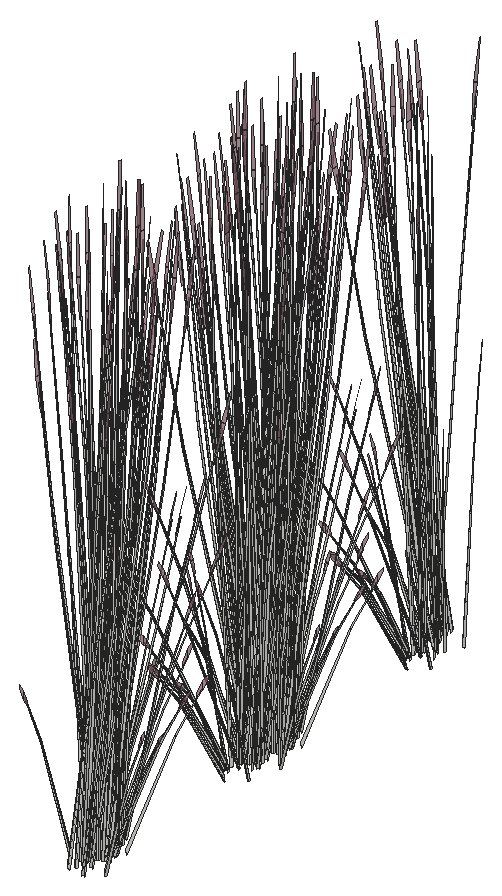
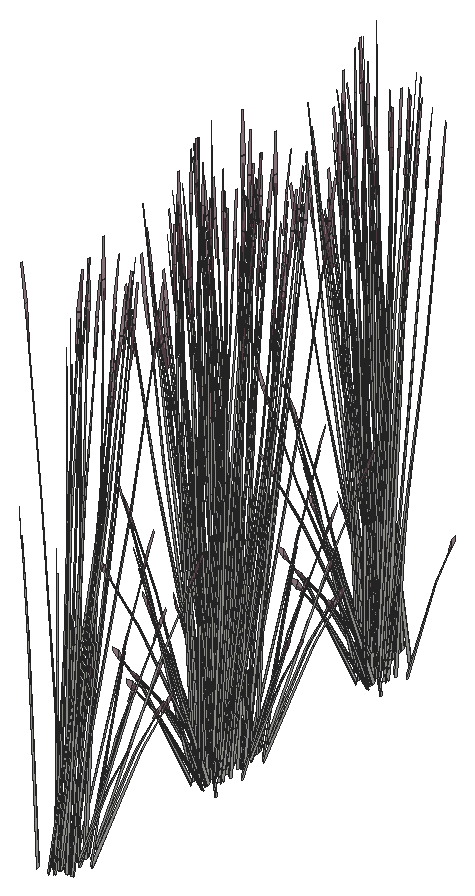
# SketchUp Ruby script. Lengths in inches.
U = 1.inch
M = Sketchup.active_model
def pt(a) = Geom::Point3d.new(a.map { |v| v * U })
def face(e, loops, mat)
  f = e.add_face(loops[0].map { |a| pt(a) })
  loops[1..].each { |l| e.add_face(l.map { |a| pt(a) }).erase! }
  f.material = f.back_material = mat if mat
  f
end
# faces: each face lists its corners as indices into pts; further lists are holes
def faces(e, pts, list, mat = nil) = list.each { |f| face(e, (f[0].is_a?(Array) ? f : [f]).map { |l| l.map { |i| pts[i] } }, mat) }
# xy, xz, yz: faces in a plane at the given z, y or x. An outline is a flat list of corners, or four numbers for a rectangle; further outlines are holes
def ring(l) = l.size == 4 ? [[l[0], l[1]], [l[2], l[1]], [l[2], l[3]], [l[0], l[3]]] : l.each_slice(2).to_a
def flat(e, list, mat, &to3) = list.each { |f| face(e, (f[0].is_a?(Array) ? f : [f]).map { |l| ring(l).map { |u, v| to3.(u, v) } }, mat) }
def xy(e, z, list, mat = nil) = flat(e, list, mat) { |x, y| [x, y, z] }
def xz(e, y, list, mat = nil) = flat(e, list, mat) { |x, z| [x, y, z] }
def yz(e, x, list, mat = nil) = flat(e, list, mat) { |y, z| [x, y, z] }
def lines(e, pts, list) = list.each { |a, b| e.add_line(pt(pts[a]), pt(pts[b])) }
# prism: a flat outline (further loops are holes) pulled along v
def prism(e, loops, v, mat = nil)
  f = face(e, loops, mat); d = Geom::Vector3d.new(v.map { |x| x * U })
  f.pushpull(f.normal.samedirection?(d) ? d.length : -d.length)
end
def box(e, o, s, mat = nil) = prism(e, [[o, [o[0] + s[0], o[1], o[2]], [o[0] + s[0], o[1] + s[1], o[2]], [o[0], o[1] + s[1], o[2]]]], [0, 0, s[2]], mat)
def at(x, y, z, deg = 0) = Geom::Transformation.translation(pt([x, y, z])) * Geom::Transformation.rotation(ORIGIN, Z_AXIS, deg.degrees)
def axes(o, x, y, z) = Geom::Transformation.new([*x, 0, *y, 0, *z, 0, *pt(o).to_a, 1])
def part(name) = M.definitions.add(name)
# library, detail: a bought-in or finely detailed component or shape, given as its bounding box
def library(name, o, s) = part(name).tap { |d| box(d.entities, o, s) }
def detail(e, o, s) = box(e.add_group.entities, o, s)
def put(e, d, t, mat = nil) = e.add_instance(d, t).tap { |i| i.material = mat if mat }
def group(e, t, mat = nil) = e.add_group.tap { |g| g.transformation = t; g.material = mat if mat }.entities
root = M.entities
M.materials.add("LightPink_Translucent").color = [144, 107, 117]
M.materials["LightPink_Translucent"].alpha = 0.75
c1 = part("blade")
p = [[2.15,0.21,22],[0,0.17,0],[0.09,0.45,0],[2.18,0.31,22],[2.29,0.31,22],[0.38,0.45,0],
  [2.48,0.24,33],[2.49,0.24,33],[2.48,0.22,33]]
faces(c1.entities,p,[[0,1,2,3],[4,5,2,3],[6,3,4,7],[8,0,3,6]])
c2 = part("seeds")
p = [[0.3,-0.1,1.38],[-0.01,-0.03,1.59],[-0.01,-0.03,0.03],[0.14,-0.07,-0.07],[0.29,-0.03,3],[0.15,0.01,3.11]]
faces(c2.entities,p,[[0,1,2,3],[1,0,4,5]],"LightPink_Translucent")
c3 = part("blade with seeds")
put(c3.entities,c1,at(0,0,0))
put(c3.entities,c2,axes([2.4,0.25,30.99],[1.5799,-0.05474,1.17369],[-0.12525,1.92788,0.29478],[-0.07173,-0.02425,1.56792]))
put(root,c3,axes([251.23,97.13,0.35],[-0.25194,0.2448,0.93574],[-0.08019,-0.7024,0.36359],[0.1547,0.01169,1.0643]))
put(root,c3,axes([251.91,97.3125,1.09],[0.04938,-0.54569,0.10509],[0.24125,0.09472,-0.30009],[0.0439,0.05603,0.91989]))
put(root,c3,axes([251.49,98.61,0.91],[0.32351,0.12883,0.33208],[-0.06584,0.72759,0.13031],[-0.04728,-0.07026,1.15295]))
put(root,c3,axes([253.2,98.08,0.28],[-0.01338,-0.09283,1.27986],[0.09278,-0.54301,-0.19552],[0.09359,-0.00781,0.218]))
put(root,c3,axes([250.44,97.99,0.28],[0.00649,0.09636,1.27986],[-0.13086,0.50324,-0.19552],[-0.09295,-0.02537,0.218]))
put(root,c3,axes([251.81,97.46,1.17],[-0.15376,-0.51322,0.32471],[0.2329,-0.3614,-0.15627],[0.04976,0.0635,1.04254]))
put(root,c3,axes([251.01,99.8,0.66],[-0.06012,-0.53279,-0.22483],[0.23879,-0.15129,0.22483],[-0.04814,-0.06144,1.00865]))
put(root,c3,axes([251.32,99.77,0.99],[0.27504,-0.16229,0.12804],[0.06792,0.60396,0.25465],[-0.02453,-0.088,1.1642]))
put(root,c3,axes([251.89,97.49,1.13],[0.25843,-0.40595,-0.21117],[0.17185,0.5736,-0.36291],[0.06376,0.05825,1.15913]))
put(root,c3,axes([250.95,100.03,0.66],[-0.23955,-0.30573,-0.36036],[0.14318,-0.54821,0],[-0.05456,-0.06963,1.14313]))
put(root,c3,axes([252.54,96.41,0.66],[0.23955,0.30573,-0.36036],[-0.14318,0.54821,0],[0.05456,0.06963,1.14313]))
put(root,c3,axes([252.08,98.16,0.79],[0.28637,0,0],[0,0.63302,0],[0,0,1.29484]))
put(root,c3,axes([251.6,98.95,1.13],[-0.25843,0.40595,-0.21117],[-0.17185,-0.5736,-0.36291],[-0.06376,-0.05825,1.15913]))
put(root,c3,axes([252.16,96.67,0.99],[-0.27504,0.16229,0.12804],[-0.06792,-0.60396,0.25465],[0.02453,0.088,1.1642]))
put(root,c3,axes([252.47,96.64,0.66],[0.06012,0.53279,-0.22483],[-0.23879,0.15129,0.22483],[0.04814,0.06144,1.00865]))
put(root,c3,axes([251.99,97.83,0.92],[-0.32351,-0.12883,0.35707],[0.06584,-0.72759,0.14012],[0.04728,0.07026,1.23973]))
put(root,c3,axes([251.73,99.63,0.79],[-0.08351,-0.52716,0],[0.23848,-0.18461,0],[0,0,1.1204]))
put(root,c3,axes([251.57,99.13,1.09],[-0.04938,0.54569,0.10509],[-0.24125,-0.09472,-0.30009],[-0.0439,-0.05603,0.91989]))
put(root,c3,axes([252.05,99.56,0.78],[0.26872,-0.20746,-0.13933],[0.09442,0.59762,0.00006],[0.02966,-0.02293,1.26212]))
put(root,c3,axes([252.14,99.8,0.99],[0.07394,-0.60768,0.12804],[0.27057,0.17197,0.25465],[-0.04674,0.00296,1.1642]))
put(root,c3,axes([252.08,98.43,0.8],[0.17867,0.39495,0],[-0.17867,0.39495,0],[0,0,1.22851]))
put(root,c3,axes([252.5625,98.25,0.99],[-0.2011,-0.44539,0.12804],[0.20266,-0.432,0.25465],[-0.02221,0.09096,1.1642]))
put(root,c3,axes([252.1875,97.58,0.6875],[0.26625,0.10025,-0.45255],[-0.05619,0.61836,-0.11877],[0.07946,0.07493,0.99892]))
put(root,c3,axes([253.36,98.66,1.2],[-0.15814,0.10094,0.83364],[0.07444,-0.41719,0.6125],[0.0839,0.02855,0.18362]))
put(root,c3,axes([251.67,99.87,0.79],[-0.25804,-0.27452,0],[0.12419,-0.5704,0],[0,0,1.1809]))
put(root,c3,axes([251.89,99.14,0.98],[-0.24993,-0.49214,-0.18284],[0.21031,-0.55263,0.40012],[-0.0673,0.05757,1.22088]))
put(root,c3,axes([251.23,100.08,0.99],[0.23955,0.30573,0.36036],[-0.14318,0.54821,0],[-0.05456,-0.06963,1.14313]))
put(root,c3,axes([252.07,97.96,1.17],[0.12419,-0.55096,0.32471],[0.25804,0.26516,-0.15627],[0,0.12701,1.04254]))
put(root,c3,axes([252.03,98.28,0.86],[0,0.70714,-0.04091],[-0.32006,0,0],[0,0.02222,1.30182]))
put(root,c3,axes([252.05,97.78,0.8],[0.15376,0.51322,-0.32471],[-0.2329,0.3614,0.15627],[0.04976,0.0635,1.04254]))
put(root,c3,axes([251.09,100.4,0.91],[-0.16003,0.61271,0],[-0.26773,-0.34169,-0.37456],[-0.06098,-0.07782,1.18819]))
put(root,c3,axes([252.73,98.27,0.99],[0,-0.61145,0.36036],[0.28637,0,0],[0,0.13926,1.14313]))
put(root,c3,axes([252.01,98.73,1.17],[0.27795,-0.03775,0.32471],[0.02514,0.62656,-0.15627],[-0.04976,0.0635,1.04254]))
put(root,c3,axes([252.18,98.09,1.09],[0.23848,-0.17832,0.10509],[0.08351,0.5092,-0.30009],[0,0.11207,0.91989]))
put(root,c3,axes([251.76,99.03,0.8],[-0.27795,0.03775,-0.32471],[-0.02514,-0.62656,0.15627],[-0.04976,0.0635,1.04254]))
put(root,c3,axes([253.07,99.33,1.07],[-0.06164,-0.15038,1.03788],[0.0802,-0.49748,-0.22321],[0.12472,0.06739,0.44375]))
put(root,c3,axes([251.97,99.88,0.79],[0.25804,0.27452,0],[-0.12419,0.5704,0],[0,0,1.26978]))
put(root,c3,axes([252.07,100.49,0.78],[-0.15803,-0.61485,-0.03732],[0.26773,-0.34169,0.37456],[-0.06597,0.05854,1.1876]))
put(root,c3,axes([252.01,99,1.09],[0.1891,0.36737,0.10509],[-0.15773,0.41447,-0.30009],[-0.0439,0.05603,0.91989]))
put(root,c3,axes([252.21,100.13,0.99],[0.23955,-0.30573,0.36036],[0.14318,0.54821,0],[-0.05456,0.06963,1.14313]))
put(root,c3,axes([251.875,99.65,0.86],[0.11128,0.70245,-0.04364],[-0.31797,0.24614,0],[0.00389,0.02453,1.2496]))
put(root,c3,axes([252,100.41,0.66],[-0.23879,-0.15129,-0.22483],[0.06012,-0.53279,0.22483],[-0.04814,0.06144,1.00865]))
put(root,c3,axes([250.27,99.33,1.07],[0.08895,0.05019,1.03788],[0.05733,0.5127,-0.22321],[-0.12083,0.09597,0.44375]))
put(root,c3,axes([252.92,98.375,0.92],[0.32006,0,0],[0,0.68339,-0.37456],[0,0.15565,1.18819]))
put(root,c3,axes([252.79,98.73,0.79],[-0.3199,-0.00489,-0.03612],[0,-0.68339,0.36248],[-0.01005,0.15557,1.14929]))
put(root,c3,axes([252.1,98.13,1.13],[0.28825,0.29175,-0.21117],[-0.1388,0.61578,-0.36291],[0.00906,0.15119,1.15913]))
put(root,c3,axes([250.09,100.4,1.2],[0.10667,-0.27712,0.83364],[0.04209,0.43871,0.6125],[-0.07709,0.07855,0.18362]))
put(root,c3,axes([252.73,98.83,0.66],[-0.17867,0.3815,-0.22483],[-0.17867,-0.3815,0.22483],[0,0.12288,1.00865]))
put(root,c3,axes([251.96,98.86,1.13],[0.02983,0.6977,-0.21117],[-0.31064,0.04219,-0.36291],[-0.0547,0.09294,1.15913]))
put(root,c3,axes([252.07,98.59,0.8],[-0.12419,0.55096,-0.32471],[-0.25804,-0.26516,0.15627],[0,0.12701,1.04254]))
put(root,c3,axes([251.77,99.4,0.6875],[-0.1724,0.45959,-0.45255],[-0.21416,-0.41674,-0.11877],[-0.06908,0.11465,0.99892]))
put(root,c3,axes([252.08,100.17,0.88],[0.32044,0.19874,0.22322],[-0.08017,0.71038,-0.26485],[-0.05304,0.08891,1.19671]))
put(root,c3,axes([252.05,100.65,0.66],[-0.23955,0.30573,-0.36036],[-0.14318,-0.54821,0],[-0.05456,0.06963,1.14313]))
put(root,c3,axes([252.85,98.84,0.66],[0,0.61145,-0.36036],[-0.28637,0,0],[0,0.13926,1.14313]))
put(root,c3,axes([252.49,100.11,1.2],[-0.14411,-0.17581,0.83364],[0.18609,-0.17864,0.6125],[0.05019,0.15132,0.18362]))
put(root,c3,axes([252.27,100.55,0.91],[0.16003,0.61271,0],[-0.26773,0.34169,-0.37456],[-0.06098,0.07782,1.18819]))
put(root,c3,axes([252.53,100.76,0.28],[0.01865,-0.08828,1.27986],[0.23477,-0.25998,-0.19552],[0.07118,0.13456,0.218]))
put(root,c3,axes([252.13,98.13,1.26],[-0.00699,-0.5757,1.02533],[0.31645,0.14923,0.43413],[-0.07484,0.31502,0.96783]))
put(root,c3,axes([252.22,98.76,0.71],[0.09385,0.55983,-0.50233],[-0.27035,0.20162,-0.13184],[0.01037,0.18957,1.1088]))
put(root,c3,axes([250.37,100.6875,0.28],[0.03433,0.06109,1.27986],[0.05822,0.56601,-0.19552],[-0.07609,0.1207,0.218]))
put(root,c3,axes([252.51,100.91,1.13],[-0.16414,-0.01918,0.76251],[0.10839,-0.40729,0.421],[0.06484,0.1447,0.59812]))
put(root,c3,axes([251.97,99.92,1.07],[0.00452,-0.20269,1.03788],[0.21585,-0.22641,-0.22321],[0.06663,0.2426,0.44375]))
put(root,c3,axes([250.99,101.61,1.2],[-0.00662,-0.36357,0.83364],[0.16552,0.25931,0.6125],[-0.03255,0.17329,0.18362]))
put(root,c3,axes([251.43,100.74,0.28],[0.04142,-0.03327,1.27986],[0.24917,0.18313,-0.19552],[0.00729,0.2064,0.218]))
put(root,c3,axes([250.86,100.82,1.24],[0.23252,-0.10828,0.04723],[0.05346,0.43623,-0.62638],[-0.01474,0.22082,0.56147]))
put(root,c3,axes([251.51,100.51,2.81],[0.12216,0.49718,-0.51563],[-0.25147,0.27708,0.06223],[0.02857,0.24022,0.72942]))
put(root,c3,axes([250.8,101.29,1.07],[0.08077,-0.09646,1.03788],[0.19942,0.29084,-0.22321],[-0.05936,0.25166,0.44375]))
put(root,c3,axes([252.15,112.15,1.07],[-0.07276,0.12376,1.03788],[-0.21789,-0.21662,-0.22321],[0.04039,-0.2694,0.44375]))
put(root,c3,axes([251.03,111.91,1.07],[-0.0155,0.20002,1.03788],[-0.22659,0.16744,-0.22321],[-0.05297,-0.25854,0.44375]))
put(root,c3,axes([251.61,111.48,0.28],[-0.04293,0.02203,1.27986],[-0.23742,-0.24798,-0.19552],[0.00398,-0.20684,0.218]))
put(root,c3,axes([251.88,111.16,1.2],[0.03283,0.35655,0.83364],[-0.18215,-0.19748,0.6125],[0.0196,-0.18257,0.18362]))
put(root,c3,axes([250.95,111.59,1.2],[0.13352,0.21281,0.83364],[-0.19445,0.12793,0.6125],[-0.0416,-0.16355,0.18362]))
put(root,c3,axes([250.84,112.23,0.28],[-0.02479,0.08055,1.27986],[-0.25056,0.17367,-0.19552],[-0.06053,-0.15798,0.218]))
put(root,c3,axes([251.25,114.45,0.72],[-0.10512,-0.62701,-0.50685],[0.30279,-0.22582,-0.13303],[-0.01162,-0.21232,1.11879]))
put(root,c3,axes([252.66,112.53,0.28],[-0.03831,-0.04817,1.27986],[-0.0984,-0.53815,-0.19552],[0.06638,-0.14604,0.218]))
put(root,c3,axes([251.21,112.64,0.91],[-0.16003,-0.61271,0],[0.26773,-0.34169,-0.37456],[0.06098,-0.07782,1.18819]))
put(root,c3,axes([251.56,111.9,0.74],[-0.17688,0.35078,-0.02825],[-0.16207,-0.38418,-0.1281],[-0.01141,-0.10886,0.42251]))
put(root,c3,axes([250.64,114.36,0.66],[0,-0.61145,-0.36036],[0.28637,0,0],[0,-0.13926,1.14313]))
put(root,c3,axes([251.43,112.55,0.66],[0.23955,-0.30573,-0.36036],[0.14318,0.54821,0],[0.05456,-0.06963,1.14313]))
put(root,c3,axes([252.85,113.6,1.07],[-0.09144,-0.01811,1.03788],[-0.09368,-0.48584,-0.22321],[0.11233,-0.13744,0.44375]))
put(root,c3,axes([251.71,113.8,0.6875],[0.1724,-0.45959,-0.45255],[0.21416,0.41674,-0.11877],[0.06908,-0.11465,0.99892]))
put(root,c3,axes([252.96,112.71,1.2],[-0.08525,0.31126,0.83364],[-0.07328,-0.41819,0.6125],[0.07041,-0.10479,0.18362]))
put(root,c3,axes([251.41,114.61,0.8],[0.12419,-0.55096,-0.32471],[0.25804,0.26516,0.15627],[0,-0.12701,1.04254]))
put(root,c3,axes([251.53,114.33,1.13],[-0.02983,-0.6977,-0.21117],[0.31064,-0.04219,-0.36291],[0.0547,-0.09294,1.15913]))
put(root,c3,axes([250.76,114.37,0.66],[0.17867,-0.3815,-0.22483],[0.17867,0.3815,0.22483],[0,-0.12288,1.00865]))
put(root,c3,axes([250.6875,112.54,0.74],[-0.07384,0.49928,-0.02825],[-0.22725,-0.15358,-0.1281],[-0.0345,-0.08166,0.42251]))
put(root,c3,axes([251.38,115.07,1.13],[-0.28825,-0.29175,-0.21117],[0.1388,-0.61578,-0.36291],[-0.00906,-0.15119,1.15913]))
put(root,c3,axes([250.5625,114.82,0.91],[-0.32006,0,0],[0,-0.68339,-0.37456],[0,-0.15565,1.18819]))
put(root,c3,axes([250.62,113.6,1.07],[0.04997,0.17024,1.03788],[-0.11515,0.46273,-0.22321],[-0.11824,-0.1106,0.44375]))
put(root,c3,axes([251.49,112.79,0.66],[0.23879,0.15129,-0.22483],[-0.06012,0.53279,0.22483],[0.04814,-0.06144,1.00865]))
put(root,c3,axes([250.8125,114.64,0.88],[-0.23808,0.51407,0.22322],[-0.23822,-0.50866,-0.26485],[-0.00831,-0.14599,1.19671]))
put(root,c3,axes([251.57,114.88,0.96],[0.28839,0.29636,0.17466],[-0.1388,0.61578,0.36291],[0,-0.14195,1.16519]))
put(root,c3,axes([251.46,115.71,0.96],[0.06784,-0.72454,-0.17004],[0.32166,0.1263,0.37211],[-0.05621,-0.10006,1.13542]))
put(root,c3,axes([250.32,114.11,1.2],[0.16341,-0.04375,0.83364],[-0.10366,0.38551,0.6125],[-0.08075,-0.05783,0.18362]))
put(root,c3,axes([251.48,114.47,1.17],[-0.27795,0.03775,0.32471],[-0.02514,-0.62656,-0.15627],[0.04976,-0.0635,1.04254]))
put(root,c3,axes([250.76,114.93,0.99],[0,0.61145,0.36036],[-0.28637,0,0],[0,-0.13926,1.14313]))
put(root,c3,axes([252.39,112.8,0.92],[0.16003,-0.61271,0],[0.26773,0.34169,-0.37456],[0.06098,0.07782,1.18819]))
put(root,c3,axes([251.43,115.42,0.8],[-0.15376,-0.51322,-0.32471],[0.2329,-0.3614,0.15627],[-0.04976,-0.0635,1.04254]))
put(root,c3,axes([251.47,114.69,0.91],[0.11128,0.68373,0.33208],[-0.31797,0.23776,0.13031],[0.00389,-0.12563,1.15295]))
put(root,c3,axes([253.02,115.22,0.63],[-0.16485,0.07338,1.02759],[-0.02624,-0.58408,0.05882],[0.11546,-0.08841,0.58473]))
put(root,c3,axes([253.32,114.7,0.83],[-0.15869,-0.39099,-0.04709],[0.1738,-0.35825,-0.21349],[0.04925,-0.02522,0.70419]))
put(root,c3,axes([251.41,115.23,1.17],[-0.12419,0.55096,0.32471],[-0.25804,-0.26516,-0.15627],[0,-0.12701,1.04254]))
put(root,c3,axes([251.87,114.75,0.79],[0,-0.70749,0],[0.32006,0,0],[0,0,1.30246]))
put(root,c3,axes([252.25,113.12,0.99],[-0.23955,-0.30573,0.36036],[0.14318,-0.54821,0],[0.05456,0.06963,1.14313]))
put(root,c3,axes([251.3,115.62,0.6875],[-0.26625,-0.10025,-0.45255],[0.05619,-0.61836,-0.11877],[-0.07946,-0.07493,0.99892]))
put(root,c3,axes([251.71,114.31,0.91],[-0.21222,0.5549,0.33208],[-0.25213,-0.48983,0.13031],[0.05116,-0.05538,1.15295]))
put(root,c3,axes([251.95,115.3,0.86],[-0.23808,-0.52628,-0.0445],[0.23822,-0.5266,0],[-0.00831,-0.01838,1.27426]))
put(root,c3,axes([251.35,113.39,0.99],[-0.07394,0.60768,0.12804],[-0.27057,-0.17197,0.25465],[0.04674,-0.00296,1.1642]))
put(root,c3,axes([251.23,113.88,0.35],[-0.25194,0.2448,0.93574],[-0.08019,-0.7024,0.36359],[0.1547,0.01169,1.0643]))
put(root,c3,axes([251.91,114.07,1.09],[0.04938,-0.54569,0.10509],[0.24125,0.09472,-0.30009],[0.0439,0.05603,0.91989]))
put(root,c3,axes([251.49,115.36,0.91],[0.32351,0.12883,0.33208],[-0.06584,0.72759,0.13031],[-0.04728,-0.07026,1.15295]))
put(root,c3,axes([253.2,114.84,0.28],[-0.01338,-0.09283,1.27986],[0.09278,-0.54301,-0.19552],[0.09359,-0.00781,0.218]))
put(root,c3,axes([250.44,114.74,0.28],[0.00649,0.09636,1.27986],[-0.13086,0.50324,-0.19552],[-0.09295,-0.02537,0.218]))
put(root,c3,axes([251.81,114.21,1.17],[-0.15376,-0.51322,0.32471],[0.2329,-0.3614,-0.15627],[0.04976,0.0635,1.04254]))
put(root,c3,axes([251.01,116.56,0.66],[-0.06012,-0.53279,-0.22483],[0.23879,-0.15129,0.22483],[-0.04814,-0.06144,1.00865]))
put(root,c3,axes([251.32,116.53,0.99],[0.27504,-0.16229,0.12804],[0.06792,0.60396,0.25465],[-0.02453,-0.088,1.1642]))
put(root,c3,axes([251.89,114.25,1.13],[0.25843,-0.40595,-0.21117],[0.17185,0.5736,-0.36291],[0.06376,0.05825,1.15913]))
put(root,c3,axes([250.95,116.79,0.66],[-0.23955,-0.30573,-0.36036],[0.14318,-0.54821,0],[-0.05456,-0.06963,1.14313]))
put(root,c3,axes([252.54,113.17,0.66],[0.23955,0.30573,-0.36036],[-0.14318,0.54821,0],[0.05456,0.06963,1.14313]))
put(root,c3,axes([252.08,114.91,0.79],[0.28637,0,0],[0,0.63302,0],[0,0,1.29484]))
put(root,c3,axes([251.6,115.71,1.13],[-0.25843,0.40595,-0.21117],[-0.17185,-0.5736,-0.36291],[-0.06376,-0.05825,1.15913]))
put(root,c3,axes([252.16,113.43,0.99],[-0.27504,0.16229,0.12804],[-0.06792,-0.60396,0.25465],[0.02453,0.088,1.1642]))
put(root,c3,axes([252.47,113.39,0.66],[0.06012,0.53279,-0.22483],[-0.23879,0.15129,0.22483],[0.04814,0.06144,1.00865]))
put(root,c3,axes([251.99,114.59,0.92],[-0.32351,-0.12883,0.35707],[0.06584,-0.72759,0.14012],[0.04728,0.07026,1.23973]))
put(root,c3,axes([251.73,116.38,0.79],[-0.08351,-0.52716,0],[0.23848,-0.18461,0],[0,0,1.1204]))
put(root,c3,axes([251.57,115.88,1.09],[-0.04938,0.54569,0.10509],[-0.24125,-0.09472,-0.30009],[-0.0439,-0.05603,0.91989]))
put(root,c3,axes([252.05,116.31,0.78],[0.26872,-0.20746,-0.13933],[0.09442,0.59762,0.00006],[0.02966,-0.02293,1.26212]))
put(root,c3,axes([252.14,116.56,0.99],[0.07394,-0.60768,0.12804],[0.27057,0.17197,0.25465],[-0.04674,0.00296,1.1642]))
put(root,c3,axes([252.08,115.18,0.8],[0.17867,0.39495,0],[-0.17867,0.39495,0],[0,0,1.22851]))
put(root,c3,axes([252.5625,115.01,0.99],[-0.2011,-0.44539,0.12804],[0.20266,-0.432,0.25465],[-0.02221,0.09096,1.1642]))
put(root,c3,axes([252.1875,114.34,0.6875],[0.26625,0.10025,-0.45255],[-0.05619,0.61836,-0.11877],[0.07946,0.07493,0.99892]))
put(root,c3,axes([253.36,115.42,1.2],[-0.15814,0.10094,0.83364],[0.07444,-0.41719,0.6125],[0.0839,0.02855,0.18362]))
put(root,c3,axes([251.67,116.625,0.79],[-0.25804,-0.27452,0],[0.12419,-0.5704,0],[0,0,1.1809]))
put(root,c3,axes([251.89,115.89,0.98],[-0.24993,-0.49214,-0.18284],[0.21031,-0.55263,0.40012],[-0.0673,0.05757,1.22088]))
put(root,c3,axes([251.23,116.84,0.99],[0.23955,0.30573,0.36036],[-0.14318,0.54821,0],[-0.05456,-0.06963,1.14313]))
put(root,c3,axes([252.07,114.72,1.17],[0.12419,-0.55096,0.32471],[0.25804,0.26516,-0.15627],[0,0.12701,1.04254]))
put(root,c3,axes([252.03,115.03,0.86],[0,0.70714,-0.04091],[-0.32006,0,0],[0,0.02222,1.30182]))
put(root,c3,axes([252.05,114.53,0.8],[0.15376,0.51322,-0.32471],[-0.2329,0.3614,0.15627],[0.04976,0.0635,1.04254]))
put(root,c3,axes([251.09,117.16,0.91],[-0.16003,0.61271,0],[-0.26773,-0.34169,-0.37456],[-0.06098,-0.07782,1.18819]))
put(root,c3,axes([252.73,115.03,0.99],[0,-0.61145,0.36036],[0.28637,0,0],[0,0.13926,1.14313]))
put(root,c3,axes([252.01,115.48,1.17],[0.27795,-0.03775,0.32471],[0.02514,0.62656,-0.15627],[-0.04976,0.0635,1.04254]))
put(root,c3,axes([252.18,114.85,1.09],[0.23848,-0.17832,0.10509],[0.08351,0.5092,-0.30009],[0,0.11207,0.91989]))
put(root,c3,axes([251.76,115.79,0.8],[-0.27795,0.03775,-0.32471],[-0.02514,-0.62656,0.15627],[-0.04976,0.0635,1.04254]))
put(root,c3,axes([253.07,116.09,1.07],[-0.06164,-0.15038,1.03788],[0.0802,-0.49748,-0.22321],[0.12472,0.06739,0.44375]))
put(root,c3,axes([251.97,116.63,0.79],[0.25804,0.27452,0],[-0.12419,0.5704,0],[0,0,1.26978]))
put(root,c3,axes([252.07,117.24,0.78],[-0.15803,-0.61485,-0.03732],[0.26773,-0.34169,0.37456],[-0.06597,0.05854,1.1876]))
put(root,c3,axes([252.01,115.75,1.09],[0.1891,0.36737,0.10509],[-0.15773,0.41447,-0.30009],[-0.0439,0.05603,0.91989]))
put(root,c3,axes([252.21,116.89,0.99],[0.23955,-0.30573,0.36036],[0.14318,0.54821,0],[-0.05456,0.06963,1.14313]))
put(root,c3,axes([251.875,116.4,0.86],[0.11128,0.70245,-0.04364],[-0.31797,0.24614,0],[0.00389,0.02453,1.2496]))
put(root,c3,axes([252,117.16,0.66],[-0.23879,-0.15129,-0.22483],[0.06012,-0.53279,0.22483],[-0.04814,0.06144,1.00865]))
put(root,c3,axes([250.27,116.08,1.07],[0.08895,0.05019,1.03788],[0.05733,0.5127,-0.22321],[-0.12083,0.09597,0.44375]))
put(root,c3,axes([252.92,115.13,0.92],[0.32006,0,0],[0,0.68339,-0.37456],[0,0.15565,1.18819]))
put(root,c3,axes([252.79,115.48,0.79],[-0.3199,-0.00489,-0.03612],[0,-0.68339,0.36248],[-0.01005,0.15557,1.14929]))
put(root,c3,axes([252.1,114.89,1.13],[0.28825,0.29175,-0.21117],[-0.1388,0.61578,-0.36291],[0.00906,0.15119,1.15913]))
put(root,c3,axes([250.09,117.16,1.2],[0.10667,-0.27712,0.83364],[0.04209,0.43871,0.6125],[-0.07709,0.07855,0.18362]))
put(root,c3,axes([252.73,115.58,0.66],[-0.17867,0.3815,-0.22483],[-0.17867,-0.3815,0.22483],[0,0.12288,1.00865]))
put(root,c3,axes([251.96,115.62,1.13],[0.02983,0.6977,-0.21117],[-0.31064,0.04219,-0.36291],[-0.0547,0.09294,1.15913]))
put(root,c3,axes([252.07,115.35,0.8],[-0.12419,0.55096,-0.32471],[-0.25804,-0.26516,0.15627],[0,0.12701,1.04254]))
put(root,c3,axes([251.77,116.15,0.6875],[-0.1724,0.45959,-0.45255],[-0.21416,-0.41674,-0.11877],[-0.06908,0.11465,0.99892]))
put(root,c3,axes([252.08,116.93,0.88],[0.32044,0.19874,0.22322],[-0.08017,0.71038,-0.26485],[-0.05304,0.08891,1.19671]))
put(root,c3,axes([252.05,117.4,0.66],[-0.23955,0.30573,-0.36036],[-0.14318,-0.54821,0],[-0.05456,0.06963,1.14313]))
put(root,c3,axes([252.85,115.59,0.66],[0,0.61145,-0.36036],[-0.28637,0,0],[0,0.13926,1.14313]))
put(root,c3,axes([252.49,116.86,1.2],[-0.14411,-0.17581,0.83364],[0.18609,-0.17864,0.6125],[0.05019,0.15132,0.18362]))
put(root,c3,axes([252.27,117.31,0.91],[0.16003,0.61271,0],[-0.26773,0.34169,-0.37456],[-0.06098,0.07782,1.18819]))
put(root,c3,axes([252.53,117.52,0.28],[0.01865,-0.08828,1.27986],[0.23477,-0.25998,-0.19552],[0.07118,0.13456,0.218]))
put(root,c3,axes([252.13,114.88,1.26],[-0.00699,-0.5757,1.02533],[0.31645,0.14923,0.43413],[-0.07484,0.31502,0.96783]))
put(root,c3,axes([252.22,115.51,0.71],[0.09385,0.55983,-0.50233],[-0.27035,0.20162,-0.13184],[0.01037,0.18957,1.1088]))
put(root,c3,axes([250.37,117.44,0.28],[0.03433,0.06109,1.27986],[0.05822,0.56601,-0.19552],[-0.07609,0.1207,0.218]))
put(root,c3,axes([252.51,117.66,1.13],[-0.16414,-0.01918,0.76251],[0.10839,-0.40729,0.421],[0.06484,0.1447,0.59812]))
put(root,c3,axes([251.97,116.68,1.07],[0.00452,-0.20269,1.03788],[0.21585,-0.22641,-0.22321],[0.06663,0.2426,0.44375]))
put(root,c3,axes([250.99,118.37,1.2],[-0.00662,-0.36357,0.83364],[0.16552,0.25931,0.6125],[-0.03255,0.17329,0.18362]))
put(root,c3,axes([251.43,117.5,0.28],[0.04142,-0.03327,1.27986],[0.24917,0.18313,-0.19552],[0.00729,0.2064,0.218]))
put(root,c3,axes([250.86,117.58,1.24],[0.23252,-0.10828,0.04723],[0.05346,0.43623,-0.62638],[-0.01474,0.22082,0.56147]))
put(root,c3,axes([250.8,118.04,1.07],[0.08077,-0.09646,1.03788],[0.19942,0.29084,-0.22321],[-0.05936,0.25166,0.44375]))
put(root,c3,axes([252.15,129.59,1.07],[-0.07276,0.12376,1.03788],[-0.21789,-0.21662,-0.22321],[0.04039,-0.2694,0.44375]))
put(root,c3,axes([251.03,129.36,1.07],[-0.0155,0.20002,1.03788],[-0.22659,0.16744,-0.22321],[-0.05297,-0.25854,0.44375]))
put(root,c3,axes([251.61,128.92,0.28],[-0.04293,0.02203,1.27986],[-0.23742,-0.24798,-0.19552],[0.00398,-0.20684,0.218]))
put(root,c3,axes([251.88,128.61,1.2],[0.03283,0.35655,0.83364],[-0.18215,-0.19748,0.6125],[0.0196,-0.18257,0.18362]))
put(root,c3,axes([250.95,129.04,1.2],[0.13352,0.21281,0.83364],[-0.19445,0.12793,0.6125],[-0.0416,-0.16355,0.18362]))
put(root,c3,axes([250.84,129.68,0.28],[-0.02479,0.08055,1.27986],[-0.25056,0.17367,-0.19552],[-0.06053,-0.15798,0.218]))
put(root,c3,axes([251.25,131.89,0.72],[-0.10512,-0.62701,-0.50685],[0.30279,-0.22582,-0.13303],[-0.01162,-0.21232,1.11879]))
put(root,c3,axes([252.66,129.98,0.28],[-0.03831,-0.04817,1.27986],[-0.0984,-0.53815,-0.19552],[0.06638,-0.14604,0.218]))
put(root,c3,axes([251.21,130.09,0.91],[-0.16003,-0.61271,0],[0.26773,-0.34169,-0.37456],[0.06098,-0.07782,1.18819]))
put(root,c3,axes([251.56,129.35,0.74],[-0.17688,0.35078,-0.02825],[-0.16207,-0.38418,-0.1281],[-0.01141,-0.10886,0.42251]))
put(root,c3,axes([250.64,131.8,0.66],[0,-0.61145,-0.36036],[0.28637,0,0],[0,-0.13926,1.14313]))
put(root,c3,axes([251.43,129.99,0.66],[0.23955,-0.30573,-0.36036],[0.14318,0.54821,0],[0.05456,-0.06963,1.14313]))
put(root,c3,axes([252.85,131.05,1.07],[-0.09144,-0.01811,1.03788],[-0.09368,-0.48584,-0.22321],[0.11233,-0.13744,0.44375]))
put(root,c3,axes([251.71,131.25,0.6875],[0.1724,-0.45959,-0.45255],[0.21416,0.41674,-0.11877],[0.06908,-0.11465,0.99892]))
put(root,c3,axes([252.96,130.16,1.2],[-0.08525,0.31126,0.83364],[-0.07328,-0.41819,0.6125],[0.07041,-0.10479,0.18362]))
put(root,c3,axes([251.41,132.05,0.8],[0.12419,-0.55096,-0.32471],[0.25804,0.26516,0.15627],[0,-0.12701,1.04254]))
put(root,c3,axes([251.53,131.78,1.13],[-0.02983,-0.6977,-0.21117],[0.31064,-0.04219,-0.36291],[0.0547,-0.09294,1.15913]))
put(root,c3,axes([250.76,131.82,0.66],[0.17867,-0.3815,-0.22483],[0.17867,0.3815,0.22483],[0,-0.12288,1.00865]))
put(root,c3,axes([250.6875,129.99,0.74],[-0.07384,0.49928,-0.02825],[-0.22725,-0.15358,-0.1281],[-0.0345,-0.08166,0.42251]))
put(root,c3,axes([251.38,132.51,1.13],[-0.28825,-0.29175,-0.21117],[0.1388,-0.61578,-0.36291],[-0.00906,-0.15119,1.15913]))
put(root,c3,axes([250.5625,132.27,0.91],[-0.32006,0,0],[0,-0.68339,-0.37456],[0,-0.15565,1.18819]))
put(root,c3,axes([250.62,131.05,1.07],[0.04997,0.17024,1.03788],[-0.11515,0.46273,-0.22321],[-0.11824,-0.1106,0.44375]))
put(root,c3,axes([251.49,130.24,0.66],[0.23879,0.15129,-0.22483],[-0.06012,0.53279,0.22483],[0.04814,-0.06144,1.00865]))
put(root,c3,axes([250.8125,132.09,0.88],[-0.23808,0.51407,0.22322],[-0.23822,-0.50866,-0.26485],[-0.00831,-0.14599,1.19671]))
put(root,c3,axes([251.57,132.33,0.96],[0.28839,0.29636,0.17466],[-0.1388,0.61578,0.36291],[0,-0.14195,1.16519]))
put(root,c3,axes([251.46,133.16,0.96],[0.06784,-0.72454,-0.17004],[0.32166,0.1263,0.37211],[-0.05621,-0.10006,1.13542]))
put(root,c3,axes([250.32,131.56,1.2],[0.16341,-0.04375,0.83364],[-0.10366,0.38551,0.6125],[-0.08075,-0.05783,0.18362]))
put(root,c3,axes([251.48,131.91,1.17],[-0.27795,0.03775,0.32471],[-0.02514,-0.62656,-0.15627],[0.04976,-0.0635,1.04254]))
put(root,c3,axes([250.76,132.37,0.99],[0,0.61145,0.36036],[-0.28637,0,0],[0,-0.13926,1.14313]))
put(root,c3,axes([252.39,130.24,0.92],[0.16003,-0.61271,0],[0.26773,0.34169,-0.37456],[0.06098,0.07782,1.18819]))
put(root,c3,axes([251.43,132.86,0.8],[-0.15376,-0.51322,-0.32471],[0.2329,-0.3614,0.15627],[-0.04976,-0.0635,1.04254]))
put(root,c3,axes([251.47,132.14,0.91],[0.11128,0.68373,0.33208],[-0.31797,0.23776,0.13031],[0.00389,-0.12563,1.15295]))
put(root,c3,axes([253.02,132.66,0.63],[-0.16485,0.07338,1.02759],[-0.02624,-0.58408,0.05882],[0.11546,-0.08841,0.58473]))
